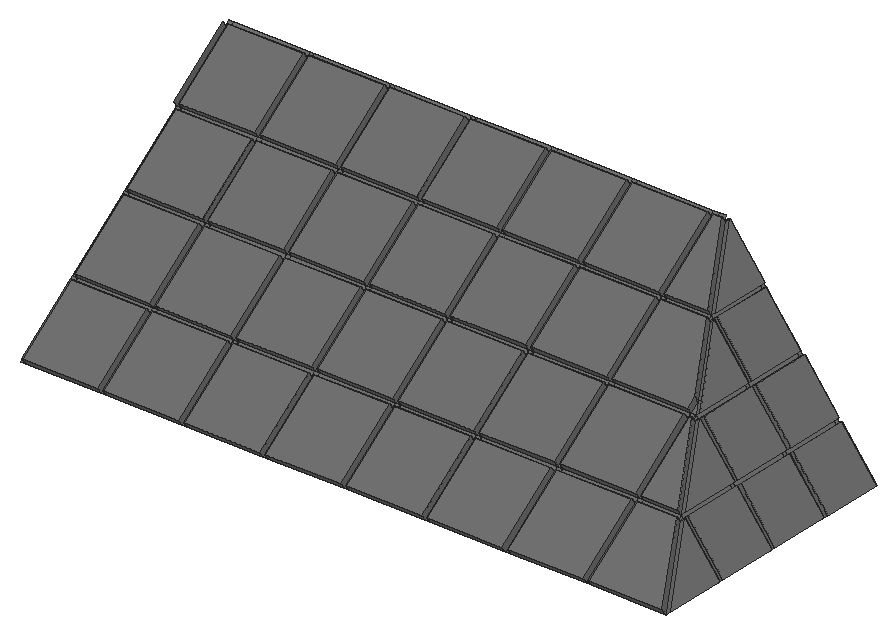
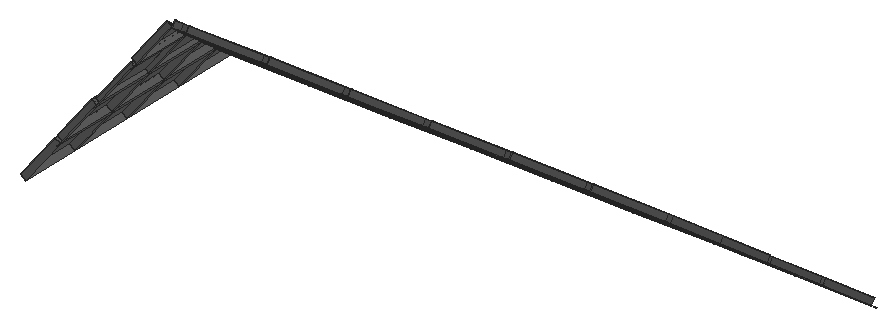
# SketchUp Ruby script. Lengths in inches.
U = 1.inch
M = Sketchup.active_model
def pt(a) = Geom::Point3d.new(a.map { |v| v * U })
def face(e, loops, mat)
  f = e.add_face(loops[0].map { |a| pt(a) })
  loops[1..].each { |l| e.add_face(l.map { |a| pt(a) }).erase! }
  f.material = f.back_material = mat if mat
  f
end
# faces: each face lists its corners as indices into pts; further lists are holes
def faces(e, pts, list, mat = nil) = list.each { |f| face(e, (f[0].is_a?(Array) ? f : [f]).map { |l| l.map { |i| pts[i] } }, mat) }
# xy, xz, yz: faces in a plane at the given z, y or x. An outline is a flat list of corners, or four numbers for a rectangle; further outlines are holes
def ring(l) = l.size == 4 ? [[l[0], l[1]], [l[2], l[1]], [l[2], l[3]], [l[0], l[3]]] : l.each_slice(2).to_a
def flat(e, list, mat, &to3) = list.each { |f| face(e, (f[0].is_a?(Array) ? f : [f]).map { |l| ring(l).map { |u, v| to3.(u, v) } }, mat) }
def xy(e, z, list, mat = nil) = flat(e, list, mat) { |x, y| [x, y, z] }
def xz(e, y, list, mat = nil) = flat(e, list, mat) { |x, z| [x, y, z] }
def yz(e, x, list, mat = nil) = flat(e, list, mat) { |y, z| [x, y, z] }
def lines(e, pts, list) = list.each { |a, b| e.add_line(pt(pts[a]), pt(pts[b])) }
# prism: a flat outline (further loops are holes) pulled along v
def prism(e, loops, v, mat = nil)
  f = face(e, loops, mat); d = Geom::Vector3d.new(v.map { |x| x * U })
  f.pushpull(f.normal.samedirection?(d) ? d.length : -d.length)
end
def box(e, o, s, mat = nil) = prism(e, [[o, [o[0] + s[0], o[1], o[2]], [o[0] + s[0], o[1] + s[1], o[2]], [o[0], o[1] + s[1], o[2]]]], [0, 0, s[2]], mat)
def at(x, y, z, deg = 0) = Geom::Transformation.translation(pt([x, y, z])) * Geom::Transformation.rotation(ORIGIN, Z_AXIS, deg.degrees)
def axes(o, x, y, z) = Geom::Transformation.new([*x, 0, *y, 0, *z, 0, *pt(o).to_a, 1])
def part(name) = M.definitions.add(name)
# library, detail: a bought-in or finely detailed component or shape, given as its bounding box
def library(name, o, s) = part(name).tap { |d| box(d.entities, o, s) }
def detail(e, o, s) = box(e.add_group.entities, o, s)
def put(e, d, t, mat = nil) = e.add_instance(d, t).tap { |i| i.material = mat if mat }
def group(e, t, mat = nil) = e.add_group.tap { |g| g.transformation = t; g.material = mat if mat }.entities
root = M.entities
M.materials.add("[Color M05]").color = [114, 114, 114]
xz(root,356.11,[[759.6,444.64,749.28,457.92,750.86,459.15,761.18,445.87]],"[Color M05]")
xz(root,357.32,[[759.6,444.64,761.18,445.87,750.86,459.15,749.28,457.92]],"[Color M05]")
xz(root,375.48,[[759.6,444.64,749.28,457.92,750.86,459.15,761.18,445.87],[748.6,458.81,738.28,472.1,739.86,473.32,750.18,460.04]],"[Color M05]")
xz(root,376.69,[[759.6,444.64,761.18,445.87,750.86,459.15,749.28,457.92],[748.6,458.81,750.18,460.04,739.86,473.32,738.28,472.1]],"[Color M05]")
xz(root,394.85,[[759.6,444.64,749.28,457.92,750.86,459.15,761.18,445.87],[748.6,458.81,738.28,472.1,739.86,473.32,750.18,460.04],[737.59,472.98,727.27,486.27,728.41,487.15,738.72,473.86]],"[Color M05]")
xz(root,396.0625,[[759.6,444.64,761.18,445.87,750.86,459.15,749.28,457.92],[748.6,458.81,750.18,460.04,739.86,473.32,738.28,472.1],[737.59,472.98,738.72,473.86,728.41,487.15,727.27,486.27]],"[Color M05]")
xz(root,414.22,[[759.6,444.64,749.28,457.92,750.86,459.15,761.18,445.87],[748.6,458.81,738.28,472.1,739.86,473.32,750.18,460.04],[737.59,472.98,727.27,486.27,728.41,487.15,738.72,473.86],[726.58,487.15,716.26,500.4375,717.84,501.67,728.16,488.38]],"[Color M05]")
yz(root,568.12,[[396.0625,487.15,414.22,500.4375,413.04,502.05,394.88,488.77]],"[Color M05]")
yz(root,569.62,[[337.95,444.64,336.77,446.25,354.93,459.54,356.11,457.92],[357.32,458.81,356.14,460.42,374.3,473.71,375.48,472.1],[376.69,472.98,375.51,474.6,393.67,487.88,394.85,486.27],[396.0625,487.15,394.88,488.77,413.04,502.05,414.22,500.4375]],"[Color M05]")
yz(root,592.12,[[337.95,444.64,356.11,457.92,354.93,459.54,336.77,446.25],[357.32,458.81,375.48,472.1,374.3,473.71,356.14,460.42],[376.69,472.98,394.85,486.27,393.67,487.88,375.51,474.6],[396.0625,487.15,414.22,500.4375,413.04,502.05,394.88,488.77]],"[Color M05]")
yz(root,593.62,[[337.95,444.64,336.77,446.25,354.93,459.54,356.11,457.92],[357.32,458.81,356.14,460.42,374.3,473.71,375.48,472.1],[376.69,472.98,375.51,474.6,393.67,487.88,394.85,486.27],[396.0625,487.15,394.88,488.77,413.04,502.05,414.22,500.4375]],"[Color M05]")
yz(root,616.13,[[396.0625,487.15,414.22,500.4375,413.04,502.05,394.88,488.77]],"[Color M05]")
yz(root,616.14,[[337.95,444.64,356.11,457.92,354.93,459.54,336.77,446.25],[357.32,458.81,375.48,472.1,374.3,473.71,356.14,460.42]],"[Color M05]")
yz(root,617.62,[[337.95,444.64,336.77,446.25,354.93,459.54,356.11,457.92],[357.32,458.81,356.14,460.42,374.3,473.71,375.48,472.1],[376.69,472.98,375.51,474.6,393.67,487.88,394.85,486.27],[396.0625,487.15,394.88,488.77,413.04,502.05,414.22,500.4375]],"[Color M05]")
yz(root,640.12,[[337.95,444.64,356.11,457.92,354.93,459.54,336.77,446.25],[357.32,458.81,375.48,472.1,374.3,473.71,356.14,460.42],[376.69,472.98,394.85,486.27,393.67,487.88,375.51,474.6],[396.0625,487.15,414.22,500.4375,413.04,502.05,394.88,488.77]],"[Color M05]")
yz(root,641.62,[[337.95,444.64,336.77,446.25,354.93,459.54,356.11,457.92],[357.32,458.81,356.14,460.42,374.3,473.71,375.48,472.1],[376.69,472.98,375.51,474.6,393.67,487.88,394.85,486.27],[396.0625,487.15,394.88,488.77,413.04,502.05,414.22,500.4375]],"[Color M05]")
yz(root,664.12,[[337.95,444.64,356.11,457.92,354.93,459.54,336.77,446.25],[357.32,458.81,375.48,472.1,374.3,473.71,356.14,460.42],[376.69,472.98,394.85,486.27,393.67,487.88,375.51,474.6],[396.0625,487.15,414.22,500.4375,413.04,502.05,394.88,488.77]],"[Color M05]")
yz(root,665.62,[[337.95,444.64,336.77,446.25,354.93,459.54,356.11,457.92],[357.32,458.81,356.14,460.42,374.3,473.71,375.48,472.1],[376.69,472.98,375.51,474.6,393.67,487.88,394.85,486.27],[396.0625,487.15,394.88,488.77,413.04,502.05,414.22,500.4375]],"[Color M05]")
yz(root,688.12,[[337.95,444.64,356.11,457.92,354.93,459.54,336.77,446.25],[357.32,458.81,375.48,472.1,374.3,473.71,356.14,460.42],[376.69,472.98,394.85,486.27,393.67,487.88,375.51,474.6],[396.0625,487.15,414.22,500.4375,413.04,502.05,394.88,488.77]],"[Color M05]")
yz(root,689.62,[[337.95,444.64,336.77,446.25,354.93,459.54,356.11,457.92],[357.32,458.81,356.14,460.42,374.3,473.71,375.48,472.1],[376.69,472.98,375.51,474.6,393.67,487.88,394.85,486.27],[396.0625,487.15,394.88,488.77,413.04,502.05,414.22,500.4375]],"[Color M05]")
yz(root,712.12,[[337.95,444.64,356.11,457.92,354.93,459.54,336.77,446.25],[357.32,458.81,375.48,472.1,374.3,473.71,356.14,460.42],[376.69,472.98,394.85,486.27,393.67,487.88,375.51,474.6],[396.0625,487.15,414.22,500.4375,413.04,502.05,394.88,488.77]],"[Color M05]")
yz(root,713.62,[[337.95,444.64,336.77,446.25,354.93,459.54,356.11,457.92],[357.32,458.81,356.14,460.42,374.3,473.71,375.48,472.1],[376.69,472.98,375.51,474.6,393.67,487.88,394.85,486.27],[396.0625,487.15,394.88,488.77,413.04,502.05,414.22,500.4375]],"[Color M05]")
yz(root,736.12,[[337.95,444.64,356.11,457.92,354.93,459.54,336.77,446.25],[357.32,458.81,375.48,472.1,374.3,473.71,356.14,460.42],[376.69,472.98,379.27,474.87,378.09,476.48,375.51,474.6]],"[Color M05]")
yz(root,737.62,[[337.95,444.64,336.77,446.25,354.93,459.54,356.11,457.92],[357.32,458.81,356.14,460.42,374.3,473.71,375.48,472.1]],"[Color M05]")
p = [[569.62,337.95,444.64],[592.12,337.95,444.64],[592.12,336.77,446.25],[569.62,336.77,446.25],[593.62,337.95,444.64],[616.14,337.95,444.64],
  [616.14,336.77,446.25],[593.62,336.77,446.25],[617.62,337.95,444.64],[640.12,337.95,444.64],[640.12,336.77,446.25],[617.62,336.77,446.25],
  [641.62,337.95,444.64],[664.12,337.95,444.64],[664.12,336.77,446.25],[641.62,336.77,446.25],[665.62,337.95,444.64],[688.12,337.95,444.64],
  [688.12,336.77,446.25],[665.62,336.77,446.25],[689.62,337.95,444.64],[712.12,337.95,444.64],[712.12,336.77,446.25],[689.62,336.77,446.25],
  [713.62,337.95,444.64],[736.12,337.95,444.64],[736.12,336.77,446.25],[713.62,336.77,446.25],[737.62,337.95,444.64],[759.6,337.95,444.64],
  [759.6,336.77,446.25],[737.62,336.77,446.25],[749.28,356.11,457.92],[749.28,354.93,459.54],[568.12,337.95,444.64],[569.62,356.11,457.92],
  [568.12,356.11,457.92],[593.62,356.11,457.92],[592.12,356.11,457.92],[617.62,356.11,457.92],[616.14,356.11,457.92],[641.62,356.11,457.92],
  [640.12,356.11,457.92],[665.62,356.11,457.92],[664.12,356.11,457.92],[689.62,356.11,457.92],[688.12,356.11,457.92],[713.62,356.11,457.92],
  [712.12,356.11,457.92],[737.62,356.11,457.92],[736.12,356.11,457.92],[761.18,337.95,445.87],[750.86,356.11,459.15],[759.6,356.11,444.64],
  [761.18,356.11,445.87],[759.6,357.32,444.64],[749.28,357.32,457.92],[759.6,375.48,444.64],[761.18,375.48,445.87],[761.18,357.32,445.87],
  [759.6,376.69,444.64],[749.28,376.69,457.92],[749.28,375.48,457.92],[759.6,394.85,444.64],[761.18,394.85,445.87],[761.18,376.69,445.87],
  [759.6,396.0625,444.64],[749.28,396.0625,457.92],[749.28,394.85,457.92],[759.6,414.22,444.64],[761.18,414.22,445.87],[761.18,396.0625,445.87],
  [750.86,375.48,459.15],[750.86,357.32,459.15],[750.86,394.85,459.15],[750.86,376.69,459.15],[750.86,414.22,459.15],[750.86,396.0625,459.15],
  [592.12,354.93,459.54],[569.62,354.93,459.54],[616.14,354.93,459.54],[593.62,354.93,459.54],[640.12,354.93,459.54],[617.62,354.93,459.54],
  [664.12,354.93,459.54],[641.62,354.93,459.54],[688.12,354.93,459.54],[665.62,354.93,459.54],[712.12,354.93,459.54],[689.62,354.93,459.54],
  [736.12,354.93,459.54],[713.62,354.93,459.54],[737.62,354.93,459.54],[569.62,357.32,458.81],[568.12,357.32,458.81],[592.12,357.32,458.81],
  [593.62,357.32,458.81],[616.14,357.32,458.81],[617.62,357.32,458.81],[640.12,357.32,458.81],[641.62,357.32,458.81],[664.12,357.32,458.81],
  [665.62,357.32,458.81],[688.12,357.32,458.81],[689.62,357.32,458.81],[712.12,357.32,458.81],[713.62,357.32,458.81],[736.12,357.32,458.81],
  [737.62,357.32,458.81],[748.6,357.32,458.81],[748.6,375.48,458.81],[748.6,376.69,458.81],[748.6,394.85,458.81],[748.6,396.0625,458.81],
  [749.28,414.22,457.92],[748.6,414.22,458.81],[749.28,415.43,457.92],[748.6,415.43,458.81],[592.12,356.14,460.42],[569.62,356.14,460.42],
  [616.14,356.14,460.42],[593.62,356.14,460.42],[640.12,356.14,460.42],[617.62,356.14,460.42],[664.12,356.14,460.42],[641.62,356.14,460.42],
  [688.12,356.14,460.42],[665.62,356.14,460.42],[712.12,356.14,460.42],[689.62,356.14,460.42],[736.12,356.14,460.42],[713.62,356.14,460.42],
  [748.6,356.14,460.42],[737.62,356.14,460.42],[738.28,375.48,472.1],[738.28,374.3,473.71],[569.62,375.48,472.1],[568.12,375.48,472.1],
  [593.62,375.48,472.1],[592.12,375.48,472.1],[617.62,375.48,472.1],[616.14,375.48,472.1],[641.62,375.48,472.1],[640.12,375.48,472.1],
  [665.62,375.48,472.1],[664.12,375.48,472.1],[689.62,375.48,472.1],[688.12,375.48,472.1],[713.62,375.48,472.1],[712.12,375.48,472.1],
  [737.62,375.48,472.1],[736.12,375.48,472.1],[750.18,357.32,460.04],[739.86,375.48,473.32],[750.18,375.48,460.04],[738.28,376.69,472.1],
  [750.18,394.85,460.04],[750.18,376.69,460.04],[738.28,396.0625,472.1],[738.28,394.85,472.1],[750.18,414.22,460.04],[750.18,396.0625,460.04],
  [738.28,415.43,472.1],[738.28,414.22,472.1],[739.86,394.85,473.32],[739.86,376.69,473.32],[739.86,414.22,473.32],[739.86,396.0625,473.32],
  [592.12,374.3,473.71],[569.62,374.3,473.71],[616.14,374.3,473.71],[593.62,374.3,473.71],[640.12,374.3,473.71],[617.62,374.3,473.71],
  [664.12,374.3,473.71],[641.62,374.3,473.71],[688.12,374.3,473.71],[665.62,374.3,473.71],[712.12,374.3,473.71],[689.62,374.3,473.71],
  [736.12,374.3,473.71],[713.62,374.3,473.71],[737.62,374.3,473.71],[569.62,376.69,472.98],[568.12,376.69,472.98],[592.12,376.69,472.98],
  [593.62,376.69,472.98],[616.14,376.69,472.98],[617.62,376.69,472.98],[640.12,376.69,472.98],[641.62,376.69,472.98],[664.12,376.69,472.98],
  [665.62,376.69,472.98],[688.12,376.69,472.98],[689.62,376.69,472.98],[712.12,376.69,472.98],[713.62,376.69,472.98],[736.12,376.69,472.98],
  [737.62,376.63,472.9375],[737.59,376.69,472.98],[737.59,394.85,472.98],[737.59,396.0625,472.98],[737.59,414.22,472.98],[737.59,415.43,472.98],
  [592.12,375.51,474.6],[569.62,375.51,474.6],[616.14,375.51,474.6],[593.62,375.51,474.6],[616.13,394.85,486.27],[616.13,393.67,487.88],
  [640.12,375.51,474.6],[617.62,375.51,474.6],[664.12,375.51,474.6],[641.62,375.51,474.6],[688.12,375.51,474.6],[665.62,375.51,474.6],
  [712.12,375.51,474.6],[689.62,375.51,474.6],[736.12,375.51,474.6],[713.62,375.51,474.6],[569.62,394.85,486.27],[568.12,394.85,486.27],
  [593.62,394.85,486.27],[592.12,394.85,486.27],[617.62,394.85,486.27],[641.62,394.85,486.27],[640.12,394.85,486.27],[665.62,394.85,486.27],
  [664.12,394.85,486.27],[689.62,394.85,486.27],[688.12,394.85,486.27],[713.62,394.85,486.27],[712.12,394.85,486.27],[736.12,379.27,474.87],
  [738.72,376.69,473.86],[737.26,379.27,475.75],[738.72,394.85,473.86],[727.27,396.0625,486.27],[727.27,394.85,486.27],[738.72,414.22,473.86],
  [738.72,396.0625,473.86],[727.27,415.43,486.27],[727.27,414.22,486.27],[728.41,394.85,487.15],[728.41,414.22,487.15],[728.41,396.0625,487.15],
  [592.12,393.67,487.88],[569.62,393.67,487.88],[593.62,393.67,487.88],[640.12,393.67,487.88],[617.62,393.67,487.88],[664.12,393.67,487.88],
  [641.62,393.67,487.88],[688.12,393.67,487.88],[665.62,393.67,487.88],[712.12,393.67,487.88],[689.62,393.67,487.88],[736.12,378.09,476.48],
  [727.27,393.67,487.88],[713.62,393.67,487.88],[569.62,396.0625,487.15],[568.12,396.0625,487.15],[592.12,396.0625,487.15],[593.62,396.0625,487.15],
  [616.13,396.0625,487.15],[617.62,396.0625,487.15],[640.12,396.0625,487.15],[641.62,396.0625,487.15],[664.12,396.0625,487.15],[665.62,396.0625,487.15],
  [688.12,396.0625,487.15],[689.62,396.0625,487.15],[712.12,396.0625,487.15],[713.62,396.0625,487.15],[726.58,396.0625,487.15],[726.58,414.22,487.15],
  [726.58,415.43,487.15],[592.12,394.88,488.77],[569.62,394.88,488.77],[616.13,394.88,488.77],[593.62,394.88,488.77],[640.12,394.88,488.77],
  [617.62,394.88,488.77],[664.12,394.88,488.77],[641.62,394.88,488.77],[688.12,394.88,488.77],[665.62,394.88,488.77],[712.12,394.88,488.77],
  [689.62,394.88,488.77],[726.58,394.88,488.77],[713.62,394.88,488.77],[716.26,414.22,500.4375],[716.26,413.04,502.05],[569.62,414.22,500.4375],
  [568.12,414.22,500.4375],[593.62,414.22,500.4375],[592.12,414.22,500.4375],[617.62,414.22,500.4375],[616.13,414.22,500.4375],[641.62,414.22,500.4375],
  [640.12,414.22,500.4375],[665.62,414.22,500.4375],[664.12,414.22,500.4375],[689.62,414.22,500.4375],[688.12,414.22,500.4375],[713.62,414.22,500.4375],
  [712.12,414.22,500.4375],[728.16,396.0625,488.38],[717.84,414.22,501.67],[728.16,414.22,488.38],[716.26,415.43,500.4375],[592.12,413.04,502.05],
  [569.62,413.04,502.05],[616.13,413.04,502.05],[593.62,413.04,502.05],[640.12,413.04,502.05],[617.62,413.04,502.05],[664.12,413.04,502.05],
  [641.62,413.04,502.05],[688.12,413.04,502.05],[665.62,413.04,502.05],[712.12,413.04,502.05],[689.62,413.04,502.05],[713.62,413.04,502.05],
  [569.62,415.43,501.32],[568.12,415.43,501.32],[592.12,415.43,501.32],[593.62,415.43,501.32],[616.13,415.43,501.32],[617.62,415.43,501.32],
  [640.12,415.43,501.32],[641.62,415.43,501.32],[664.12,415.43,501.32],[665.62,415.43,501.32],[688.12,415.43,501.32],[689.62,415.43,501.32],
  [712.12,415.43,501.32],[713.62,415.43,501.32],[715.58,415.43,501.32]]
faces(root,p,[[0,1,2,3],[4,5,6,7],[8,9,10,11],[12,13,14,15],[16,17,18,19],[20,21,22,23],[24,25,26,27],[28,29,30,31],
  [29,32,33,30],[34,0,35,36],[1,4,37,38],[5,8,39,40],[9,12,41,42],[13,16,43,44],[17,20,45,46],[21,24,47,48],
  [25,28,49,50],[32,29,51,52],[29,53,54,51],[55,56,32,53],[55,57,58,59],[60,61,62,57],[60,63,64,65],[63,66,67,68],
  [66,69,70,71],[52,51,54],[58,72,73,59],[65,64,74,75],[71,70,76,77],[3,2,78,79],[7,6,80,81],[11,10,82,83],
  [15,14,84,85],[19,18,86,87],[23,22,88,89],[27,26,90,91],[33,92,31,30],[38,35,79,78],[40,37,81,80],[42,39,83,82],
  [44,41,85,84],[46,43,87,86],[48,45,89,88],[50,47,91,90],[32,49,92,33],[36,35,93,94],[35,38,95,93],[38,37,96,95],
  [37,40,97,96],[40,39,98,97],[39,42,99,98],[42,41,100,99],[41,44,101,100],[44,43,102,101],[43,46,103,102],[46,45,104,103],
  [45,48,105,104],[48,47,106,105],[47,50,107,106],[50,49,108,107],[109,108,49,32],[109,32,56],[62,110,109,56],[62,56,73,72],
  [61,111,110,62],[61,68,112,111],[68,61,75,74],[68,67,113,112],[67,114,115,113],[114,67,77,76],[114,116,117,115],[93,95,118,119],
  [96,97,120,121],[98,99,122,123],[100,101,124,125],[102,103,126,127],[104,105,128,129],[106,107,130,131],[108,109,132,133],[109,134,135,132],
  [94,93,136,137],[95,96,138,139],[97,98,140,141],[99,100,142,143],[101,102,144,145],[103,104,146,147],[105,106,148,149],[107,108,150,151],
  [134,109,152,153],[109,110,154,152],[111,155,134,110],[111,112,156,157],[112,113,158,159],[113,115,160,161],[115,117,162,163],[153,152,154],
  [157,156,164,165],[161,160,166,167],[119,118,168,169],[121,120,170,171],[123,122,172,173],[125,124,174,175],[127,126,176,177],[129,128,178,179],
  [131,130,180,181],[135,182,133,132],[139,136,169,168],[141,138,171,170],[143,140,173,172],[145,142,175,174],[147,144,177,176],[149,146,179,178],
  [151,148,181,180],[134,150,182,135],[137,136,183,184],[136,139,185,183],[139,138,186,185],[138,141,187,186],[141,140,188,187],[140,143,189,188],
  [143,142,190,189],[142,145,191,190],[145,144,192,191],[144,147,193,192],[147,146,194,193],[146,149,195,194],[149,148,196,195],[148,151,197,196],
  [151,150,198,199,197],[134,198,150],[198,134,155,199],[155,159,200,199],[159,155,165,164],[159,158,201,200],[158,163,202,201],[163,158,167,166],
  [163,162,203,202],[183,185,204,205],[186,187,206,207],[187,208,209,206],[188,189,210,211],[190,191,212,213],[192,193,214,215],[194,195,216,217],
  [196,197,218,219],[184,183,220,221],[185,186,222,223],[187,188,224,208],[189,190,225,226],[191,192,227,228],[193,194,229,230],[195,196,231,232],
  [199,233,197],[233,199,234,235],[199,200,236,234],[200,201,237,238],[201,202,239,240],[202,203,241,242],[234,236,243,235],[240,239,244,245],
  [205,204,246,247],[207,206,209,248],[211,210,249,250],[213,212,251,252],[215,214,253,254],[217,216,255,256],[219,218,257,258,259],[233,238,258,257],
  [238,233,235,243],[223,220,247,246],[208,222,248,209],[226,224,250,249],[228,225,252,251],[230,227,254,253],[232,229,256,255],[238,231,259,258],
  [221,220,260,261],[220,223,262,260],[223,222,263,262],[222,208,264,263],[208,224,265,264],[224,226,266,265],[226,225,267,266],[225,228,268,267],
  [228,227,269,268],[227,230,270,269],[230,229,271,270],[229,232,272,271],[232,231,273,272],[274,273,231,238],[238,237,274],[237,242,275,274],
  [242,237,245,244],[242,241,276,275],[260,262,277,278],[263,264,279,280],[265,266,281,282],[267,268,283,284],[269,270,285,286],[271,272,287,288],
  [273,274,289,290],[274,291,292,289],[261,260,293,294],[262,263,295,296],[264,265,297,298],[266,267,299,300],[268,269,301,302],[270,271,303,304],
  [272,273,305,306],[291,274,307,308],[274,275,309,307],[275,276,310,291],[307,309,308],[278,277,311,312],[280,279,313,314],[282,281,315,316],
  [284,283,317,318],[286,285,319,320],[288,287,321,322],[292,323,290,289],[296,293,312,311],[298,295,314,313],[300,297,316,315],[302,299,318,317],
  [304,301,320,319],[306,303,322,321],[291,305,323,292],[294,293,324,325],[293,296,326,324],[296,295,327,326],[295,298,328,327],[298,297,329,328],
  [297,300,330,329],[300,299,331,330],[299,302,332,331],[302,301,333,332],[301,304,334,333],[304,303,335,334],[303,306,336,335],[306,305,337,336],
  [338,337,305,291]],"[Color M05]")
